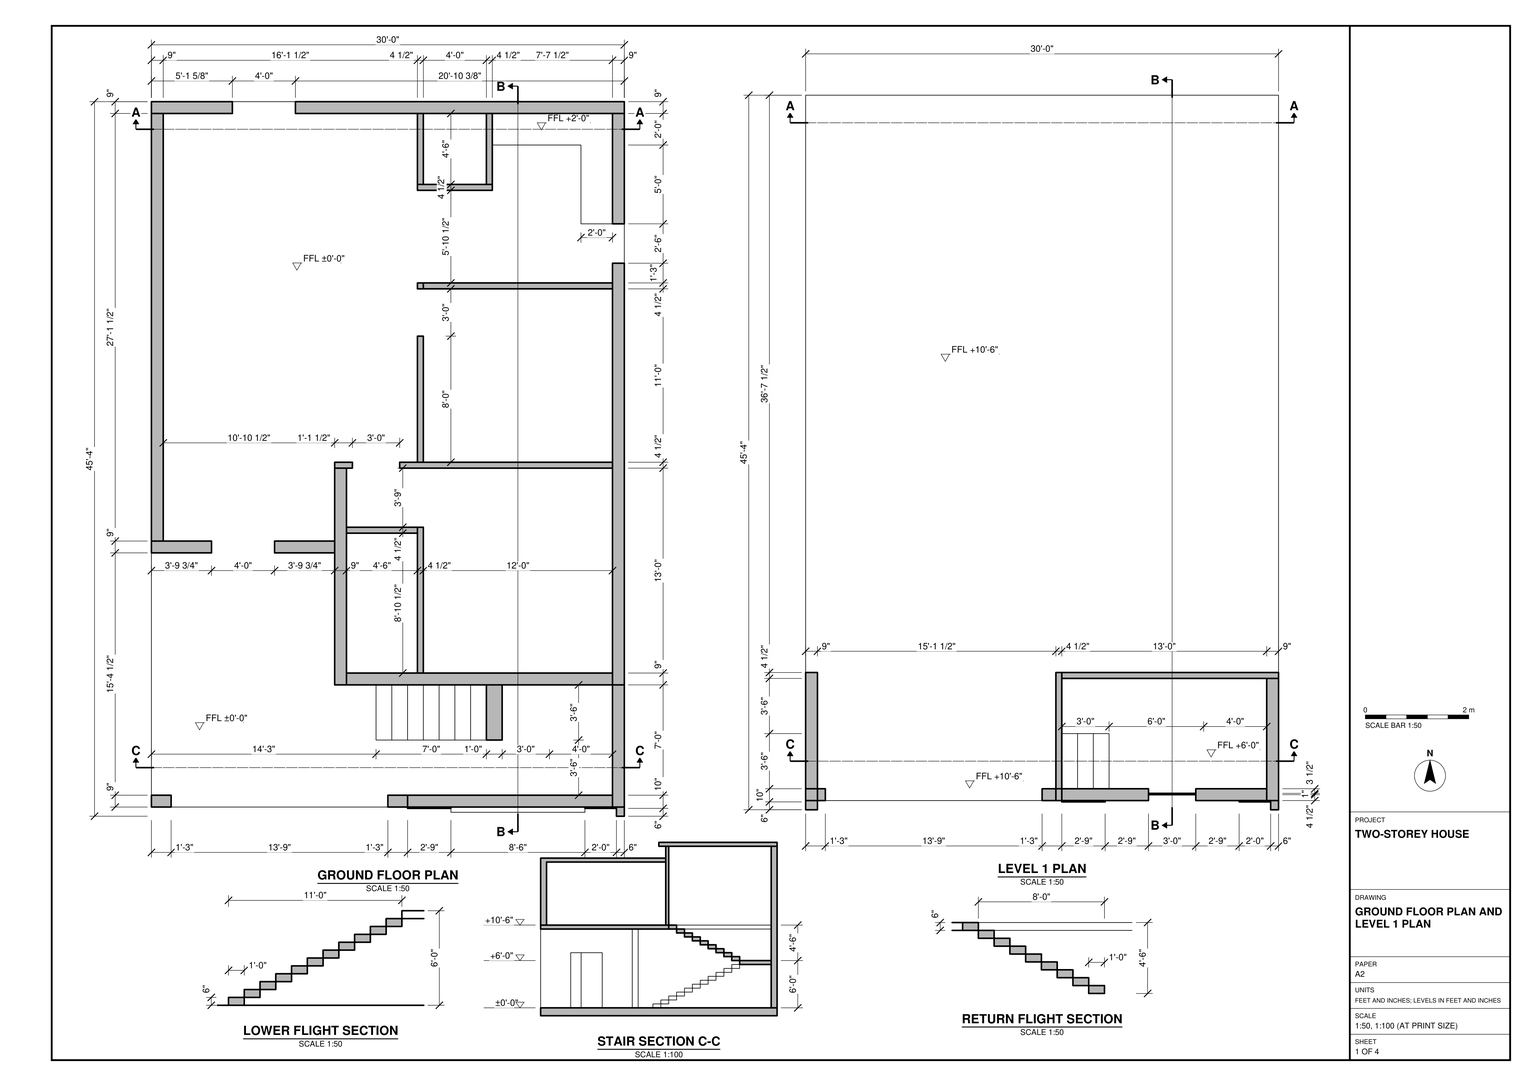
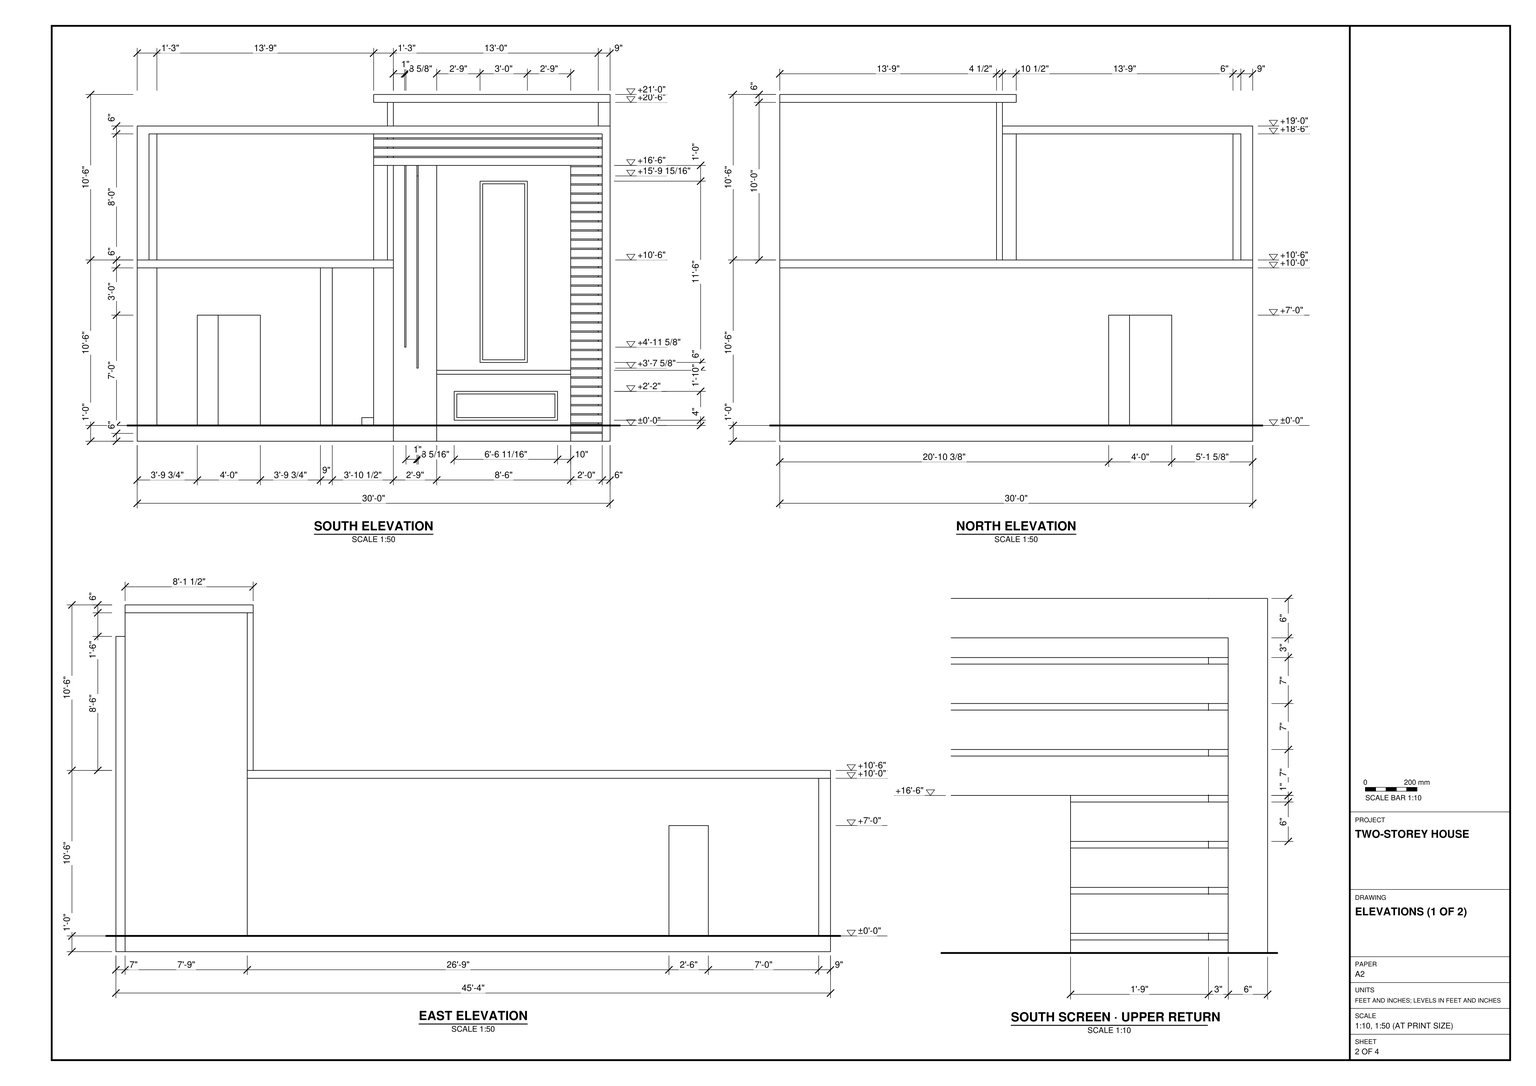
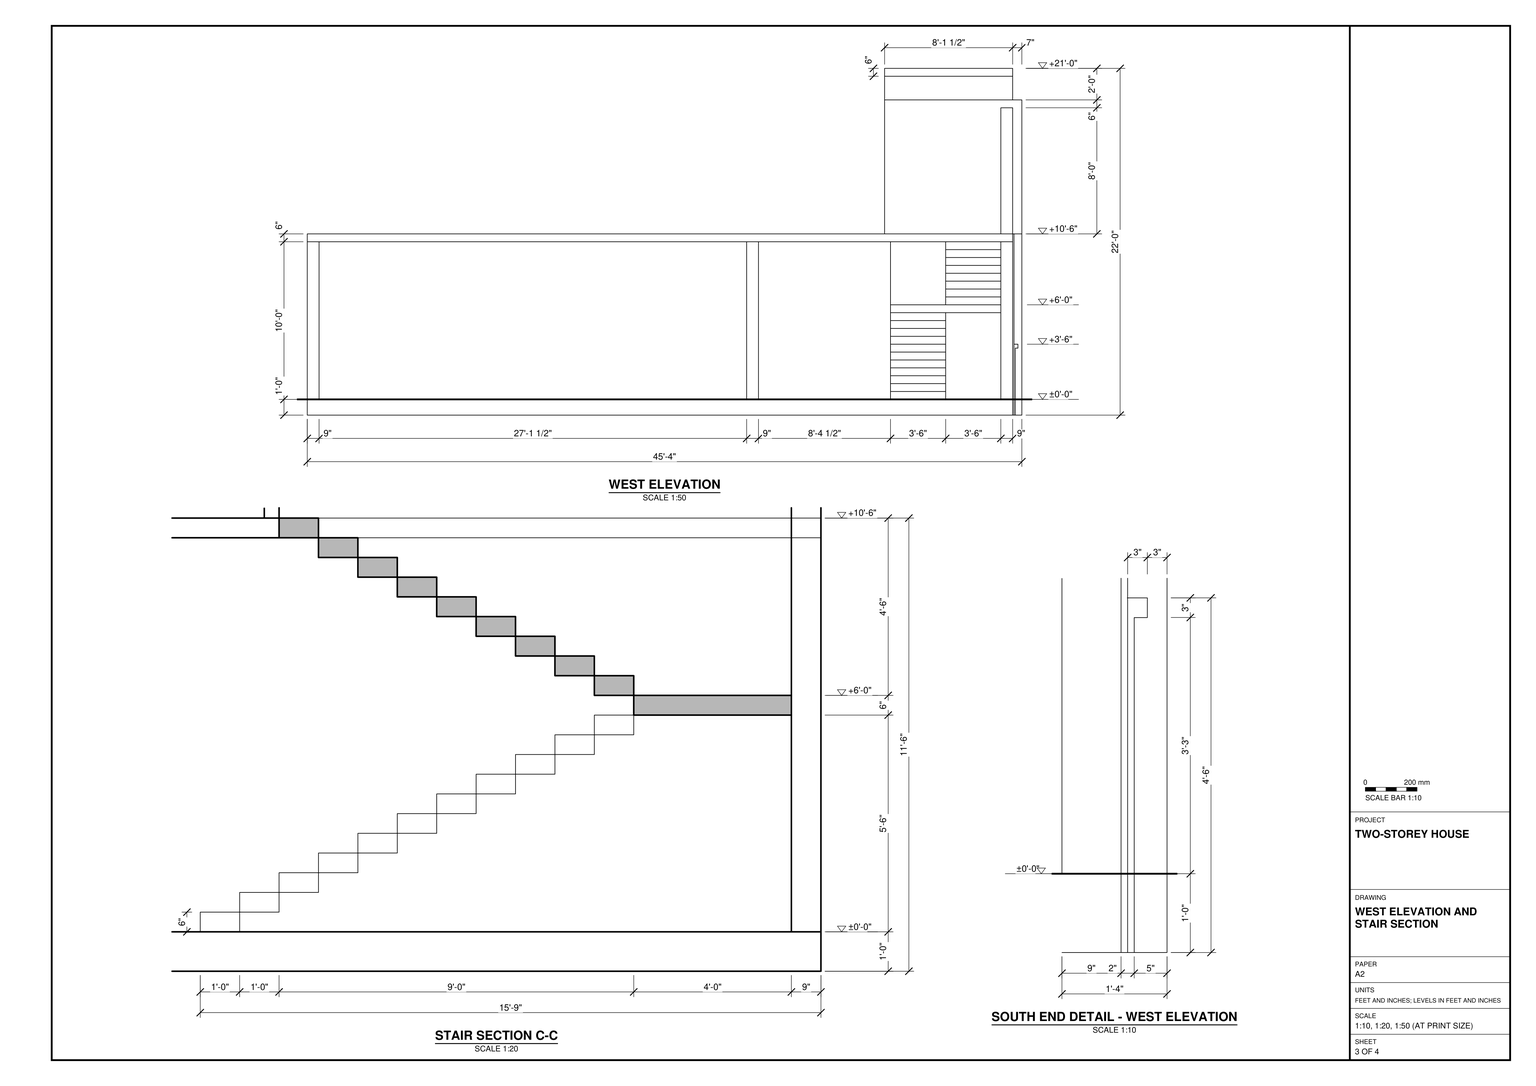
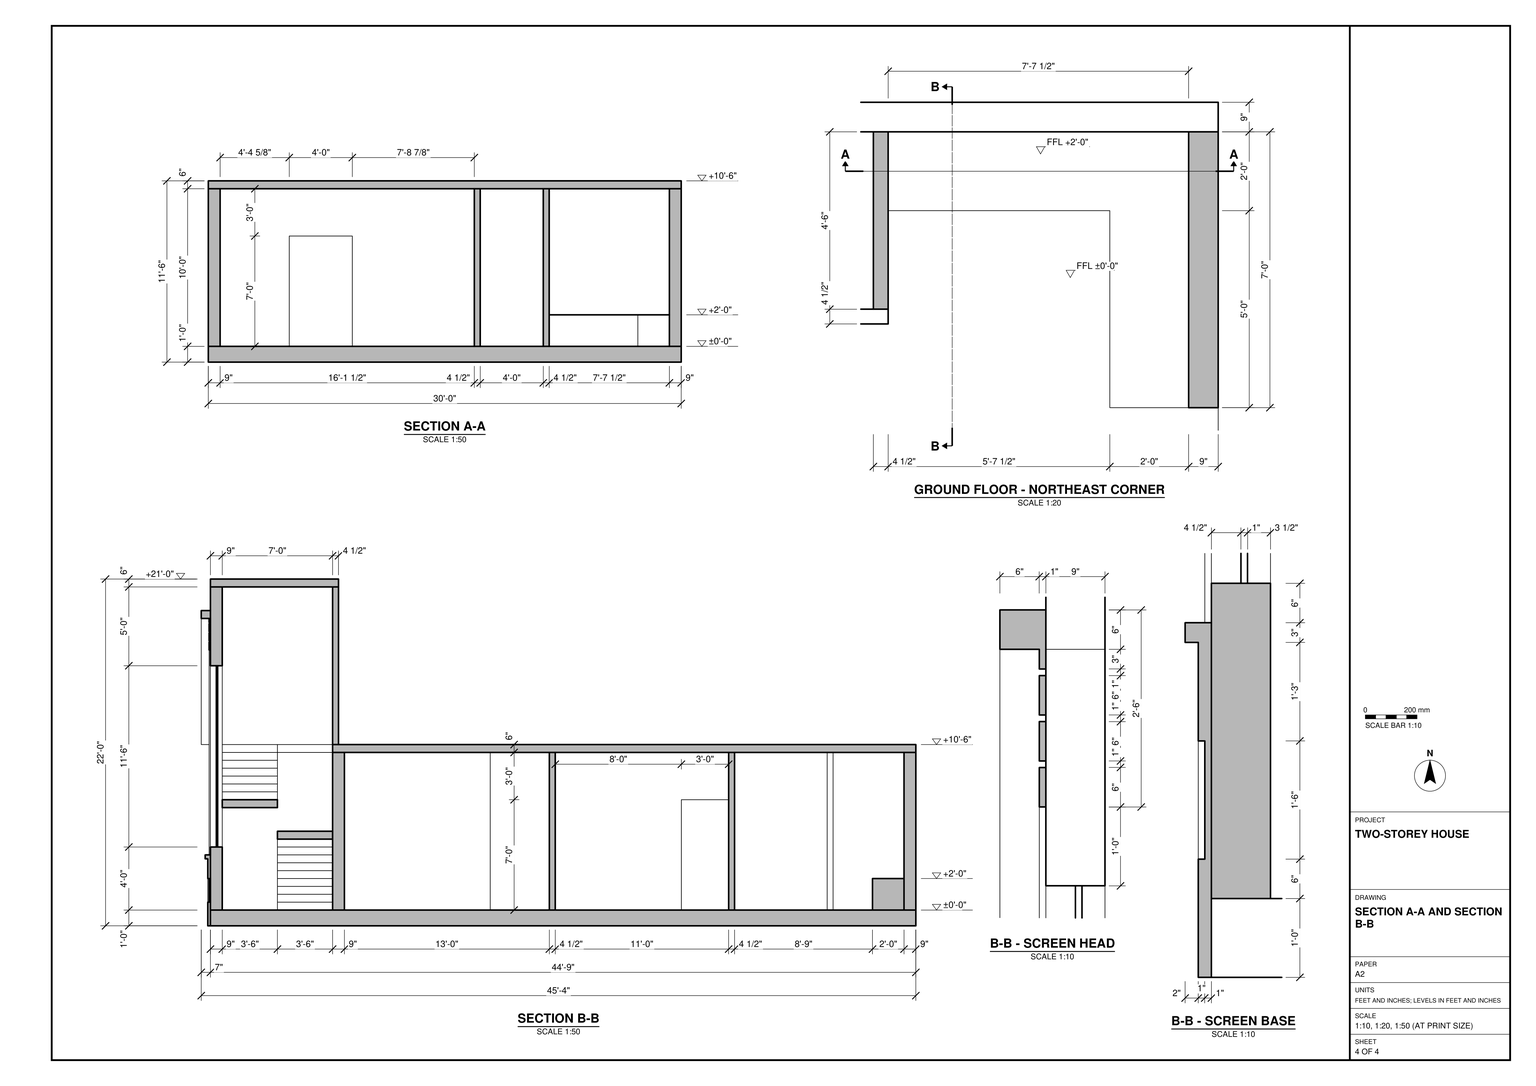
Build the house in SketchUp using task_files/diagram_01.pdf. Work in feet and inches. The house is 30'-0" wide from east to west, 45'-4" deep from north to south and 22'-0" high from the underside of the base slab to the highest roof. Set the ground floor at ±0'-0" and Level 1 at +10'-6".

Follow the ground-floor plan for the recessed south entrance, the large open floor area on the west and the partitions on the east. Use the wall thicknesses shown, distinguishing the 9" walls from the 4 1/2" partitions. Place the door openings at the offsets shown in plan and use the elevations for their heights. Model the base slab and the Level 1 slab, leaving the stair opening at the south end. Build the lower flight up to the +6'-0" landing and reverse direction for the flight to Level 1.

Keep the broad rear portion of Level 1 open and model the stepped flat roofs over the south end. Follow the south elevation for the open bay, the tall narrow frame above the low horizontal panel and the slatted screen that runs up the east edge and across the top. Keep walls, slabs, roofs, and any furniture or joinery pieces in separate groups or components; use components for repeated parts such as screen slats. Any decor or loose items may be suitable library components. Save one SketchUp model as output_files/two_storey_house_with_a_return_stair_and_south_screen.skp.

# SketchUp Ruby script. Lengths in inches.
U = 1.inch
M = Sketchup.active_model
def pt(a) = Geom::Point3d.new(a.map { |v| v * U })
def face(e, loops, mat)
  f = e.add_face(loops[0].map { |a| pt(a) })
  loops[1..].each { |l| e.add_face(l.map { |a| pt(a) }).erase! }
  f.material = f.back_material = mat if mat
  f
end
# faces: each face lists its corners as indices into pts; further lists are holes
def faces(e, pts, list, mat = nil) = list.each { |f| face(e, (f[0].is_a?(Array) ? f : [f]).map { |l| l.map { |i| pts[i] } }, mat) }
# xy, xz, yz: faces in a plane at the given z, y or x. An outline is a flat list of corners, or four numbers for a rectangle; further outlines are holes
def ring(l) = l.size == 4 ? [[l[0], l[1]], [l[2], l[1]], [l[2], l[3]], [l[0], l[3]]] : l.each_slice(2).to_a
def flat(e, list, mat, &to3) = list.each { |f| face(e, (f[0].is_a?(Array) ? f : [f]).map { |l| ring(l).map { |u, v| to3.(u, v) } }, mat) }
def xy(e, z, list, mat = nil) = flat(e, list, mat) { |x, y| [x, y, z] }
def xz(e, y, list, mat = nil) = flat(e, list, mat) { |x, z| [x, y, z] }
def yz(e, x, list, mat = nil) = flat(e, list, mat) { |y, z| [x, y, z] }
def lines(e, pts, list) = list.each { |a, b| e.add_line(pt(pts[a]), pt(pts[b])) }
# prism: a flat outline (further loops are holes) pulled along v
def prism(e, loops, v, mat = nil)
  f = face(e, loops, mat); d = Geom::Vector3d.new(v.map { |x| x * U })
  f.pushpull(f.normal.samedirection?(d) ? d.length : -d.length)
end
def box(e, o, s, mat = nil) = prism(e, [[o, [o[0] + s[0], o[1], o[2]], [o[0] + s[0], o[1] + s[1], o[2]], [o[0], o[1] + s[1], o[2]]]], [0, 0, s[2]], mat)
def at(x, y, z, deg = 0) = Geom::Transformation.translation(pt([x, y, z])) * Geom::Transformation.rotation(ORIGIN, Z_AXIS, deg.degrees)
def axes(o, x, y, z) = Geom::Transformation.new([*x, 0, *y, 0, *z, 0, *pt(o).to_a, 1])
def part(name) = M.definitions.add(name)
# library, detail: a bought-in or finely detailed component or shape, given as its bounding box
def library(name, o, s) = part(name).tap { |d| box(d.entities, o, s) }
def detail(e, o, s) = box(e.add_group.entities, o, s)
def put(e, d, t, mat = nil) = e.add_instance(d, t).tap { |i| i.material = mat if mat }
def group(e, t, mat = nil) = e.add_group.tap { |g| g.transformation = t; g.material = mat if mat }.entities
root = M.entities
M.materials.add("[Color C07]").color = [153, 76, 0]
M.materials.add("[Color E02]").color = [255, 255, 153]
M.materials.add("[Color M00]").color = [255, 255, 255]
M.materials.add("[Color M02]").color = [198, 198, 198]
M.materials.add("[Color M04]").color = [142, 142, 142]
M.materials.add("[Translucent Glass Gray]").color = [128, 128, 128]
M.materials["[Translucent Glass Gray]"].alpha = 0.5
c1 = part("Group\#30")
box(c1.entities,[0,0,0],[15,9,120])
c2 = part("Group\#22")
box(c2.entities,[0,0,0],[12,48,6])
c3 = part("Group\#25")
box(c3.entities,[0,0,0],[12,48,6])
c4 = part("Group\#23")
box(c4.entities,[0,0,0],[12,42,6])
g1 = group(root,at(0,0,-12))
g2 = group(g1,at(0,100,12),"[Color M02]")
box(g2,[0,109.5,0],[9,325.5,120])
g3 = group(g1,at(214.5,401.5,12))
box(g3,[-7.5,0,0],[144,4.5,120])
g4 = group(g1,at(202.5,481,12,-90))
box(g4,[0,0,0],[4.5,57,120])
g5 = group(g1,at(202.5,109,12))
box(g5,[0,0,0],[4.5,111,120])
g6 = group(g1,at(195,6,0),"[Color C07]")
xy(g6,0,[[0,0,33,1]])
xy(g6,210,[[0,0,33,1]])
xz(g6,0,[[0,0,33,0,33,210,18.93,210,18.93,55.65,17.93,55.65,17.93,210,9.62,210,9.62,71.625,8.62,71.625,8.62,210,0,210]])
xz(g6,0,[[17.93,55.65,18.93,201.97],[8.62,71.625,9.62,210],[17.93,201.97,18.93,210]],"[Color M00]")
xz(g6,1,[[0,0,33,210]])
yz(g6,0,[[0,0,1,210]])
yz(g6,33,[[0,0,1,210]])
g7 = group(g1,at(0,100,132),"[Color M02]")
prism(g7,[[[360,444,0],[360,0,0],[195,0,0],[195,-93,0],[0,-93,0],[0,444,0]]],[0,0,6])
g8 = group(g1,at(259.5,451,12))
xy(g8,24,[[67.5,0,91.5,0,91.5,84,0,84,0,60,67.5,60]])
xz(g8,0,[[67.5,0,91.5,24]])
xz(g8,60,[[0,0,67.5,24]])
xz(g8,84,[[0,0,67.5,24],[67.5,0,91.5,24]])
yz(g8,0,[[60,0,84,24]])
yz(g8,67.5,[[0,0,60,24]])
yz(g8,91.5,[[0,0,60,24],[60,0,84,24]])
put(g1,c1,at(0,7,12),"[Color M02]")
g9 = group(g1,at(202.5,269.5,12))
prism(g9,[[[4.5,132,0],[4.5,136.5,0],[4.5,136.5,120],[4.5,0,120],[4.5,0,0],[4.5,96,0],[4.5,96,84],[4.5,132,84]]],[-4.5,0,0])
g10 = group(g1,at(202.5,481,12))
box(g10,[0,0,0],[4.5,54,120])
g11 = group(g1,at(180,7,138),"[Color M02]")
box(g11,[0,0,0],[15,9,96])
g12 = group(g1,at(255,481,12))
box(g12,[0,0,0],[4.5,54,120])
g13 = group(g1,at(139.5,7,12),"[Color M02]")
xy(g13,0,[[55.5,0,211.5,9]])
xy(g13,48,[[121.5,0,157.5,9]])
xy(g13,186,[[121.5,0,157.5,9]])
xy(g13,246,[[55.5,0,211.5,9]])
xz(g13,0,[[[55.5,0,211.5,246],[88.5,42,190.5,198]]])
xz(g13,0,[[[88.5,42,190.5,198],[121.5,48,157.5,186]]],"[Color M04]")
xz(g13,9,[[[55.5,0,211.5,246],[121.5,48,157.5,186]]])
yz(g13,55.5,[[0,0,9,246]])
yz(g13,121.5,[[0,48,9,186]])
yz(g13,157.5,[[0,48,9,186]])
yz(g13,211.5,[[0,0,9,246]])
g14 = group(g13,at(-17.52,4.5,48))
xy(g14,0,[[139.02,0,175.02,1]])
xy(g14,138,[[139.02,0,175.02,1]])
xz(g14,0,[[[139.02,0,175.02,138],[141.02,2,173.02,136]]])
xz(g14,0,[[141.02,2,173.02,136]],"[Translucent Glass Gray]")
xz(g14,1,[[[139.02,0,175.02,138],[141.02,2,173.02,136]]])
xz(g14,1,[[141.02,2,173.02,136]],"[Translucent Glass Gray]")
yz(g14,139.02,[[0,0,1,138]])
yz(g14,175.02,[[0,0,1,138]])
g15 = group(g1,at(228,3,0),"[Color M02]")
g16 = group(g15,at(0,0,0))
xy(g16,0,[[0,2,102,4]])
xy(g16,18,[[15.31,2,90,3]])
xy(g16,36,[[15.31,2,90,3]])
xy(g16,51,[[0,0,102,2]])
xy(g16,54,[[0,0,102,4]],"[Color M00]")
xz(g16,0,[[0,51,102,54]],"[Color M00]")
xz(g16,2,[[[13.31,16,92,38],[15.31,18,90,36]]],"[Color M00]")
xz(g16,2,[[[0,0,102,51],[13.31,16,92,38]]],"[Color M04]")
xz(g16,3,[[15.31,18,90,36]],"[Color C07]")
xz(g16,4,[[0,0,102,54]])
yz(g16,0,[[2,0,2,51,0,51,0,54,4,54,4,0]])
yz(g16,15.31,[[2,18,3,36]])
yz(g16,90,[[2,18,3,36]])
yz(g16,102,[[2,0,4,0,4,54,0,54,0,51,2,51]])
g17 = group(g1,at(330,6,0),"[Color M02]")
xy(g17,0,[[24,-6,24,0,0,0,0,1,30,1,30,-6]])
xy(g17,6,[[0,0,24,1]])
xy(g17,7,[[0,0,24,1]])
xy(g17,13,[[0,0,24,1]])
xy(g17,14,[[0,0,24,1]])
xy(g17,20,[[0,0,24,1]])
xy(g17,21,[[0,0,24,1]])
xy(g17,27,[[0,0,24,1]])
xy(g17,28,[[0,0,24,1]])
xy(g17,34,[[0,0,24,1]])
xy(g17,35,[[0,0,24,1]])
xy(g17,41,[[0,0,24,1]])
xy(g17,42,[[0,0,24,1]])
xy(g17,48,[[0,0,24,1]])
xy(g17,49,[[0,0,24,1]])
xy(g17,55,[[0,0,24,1]])
xy(g17,56,[[0,0,24,1]])
xy(g17,62,[[0,0,24,1]])
xy(g17,63,[[0,0,24,1]])
xy(g17,69,[[0,0,24,1]])
xy(g17,70,[[0,0,24,1]])
xy(g17,76,[[0,0,24,1]])
xy(g17,77,[[0,0,24,1]])
xy(g17,83,[[0,0,24,1]])
xy(g17,84,[[0,0,24,1]])
xy(g17,90,[[0,0,24,1]])
xy(g17,91,[[0,0,24,1]])
xy(g17,97,[[0,0,24,1]])
xy(g17,98,[[0,0,24,1]])
xy(g17,104,[[0,0,24,1]])
xy(g17,105,[[0,0,24,1]])
xy(g17,111,[[0,0,24,1]])
xy(g17,112,[[0,0,24,1]])
xy(g17,118,[[0,0,24,1]])
xy(g17,119,[[0,0,24,1]])
xy(g17,125,[[0,0,24,1]])
xy(g17,126,[[0,0,24,1]])
xy(g17,132,[[0,0,24,1]])
xy(g17,133,[[0,0,24,1]])
xy(g17,138,[[-330,-6,-321,98.5]])
xy(g17,139,[[0,0,24,1]])
xy(g17,140,[[0,0,24,1]])
xy(g17,146,[[0,0,24,1]])
xy(g17,147,[[0,0,24,1]])
xy(g17,153,[[0,0,24,1]])
xy(g17,154,[[0,0,24,1]])
xy(g17,160,[[0,0,24,1]])
xy(g17,161,[[0,0,24,1]])
xy(g17,167,[[0,0,24,1]])
xy(g17,168,[[0,0,24,1]])
xy(g17,174,[[0,0,24,1]])
xy(g17,175,[[0,0,24,1]])
xy(g17,181,[[0,0,24,1]])
xy(g17,182,[[0,0,24,1]])
xy(g17,188,[[0,0,24,1]])
xy(g17,189,[[0,0,24,1]])
xy(g17,195,[[0,0,24,1]])
xy(g17,196,[[0,0,24,1]])
xy(g17,202,[[0,0,24,1]])
xy(g17,203,[[0,0,24,1]],"[Color E02]")
xy(g17,209,[[0,0,24,1]])
xy(g17,210,[[-150,0,0,1],[0,0,24,1]])
xy(g17,216,[[-150,0,24,1]])
xy(g17,217,[[-150,0,24,1]])
xy(g17,223,[[-150,0,24,1]])
xy(g17,224,[[-150,0,24,1]])
xy(g17,230,[[-150,0,24,1]])
xy(g17,231,[[-150,0,24,1]])
xy(g17,234,[[-321,-6,-321,98.5,-150,98.5,-150,0,24,0,24,-6],[-150,1,-139.5,98.5]])
xy(g17,240,[[-330,-6,30,-6,30,1,-139.5,1,-139.5,98.5,-330,98.5]])
xz(g17,-6,[[24,0,30,0,30,240,-330,240,-330,138,-321,138,-321,234,24,234]])
xz(g17,0,[[0,0,24,6],[0,7,24,13],[0,14,24,20],[0,21,24,27],[0,28,24,34],
  [0,35,24,41],[0,42,24,48],[0,49,24,55],[0,56,24,62],[0,63,24,69],
  [0,70,24,76],[0,77,24,83],[0,84,24,90],[0,91,24,97],[0,98,24,104],
  [0,105,24,111],[0,112,24,118],[0,119,24,125],[0,126,24,132],[0,133,24,139],
  [0,140,24,146],[0,147,24,153],[0,154,24,160],[0,161,24,167],[0,168,24,174],
  [0,175,24,181],[0,182,24,188],[0,189,24,195],[0,196,24,202],[0,203,24,209],
  [-150,210,24,216],[-150,217,24,223],[-150,224,24,230],[-150,231,24,234]],"[Color E02]")
xz(g17,1,[[0,0,0,6,24,6,24,7,0,7,0,13,24,13,24,14,0,14,0,20,24,20,24,21,0,21,0,27,24,27,24,28,0,28,0,34,24,34,24,35,0,35,0,41,24,41,24,42,0,42,0,48,24,48,24,49,0,49,0,55,24,55,24,56,0,56,0,62,24,62,24,63,0,63,0,69,24,69,24,70,0,70,0,76,24,76,24,77,0,77,0,83,24,83,24,84,0,84,0,90,24,90,24,91,0,91,0,97,24,97,24,98,0,98,0,104,24,104,24,105,0,105,0,111,24,111,24,112,0,112,0,118,24,118,24,119,0,119,0,125,24,125,24,126,0,126,0,132,24,132,24,133,0,133,0,139,24,139,24,140,0,140,0,146,24,146,24,147,0,147,0,153,24,153,24,154,0,154,0,160,24,160,24,161,0,161,0,167,24,167,24,168,0,168,0,174,24,174,24,175,0,175,0,181,24,181,24,182,0,182,0,188,24,188,24,189,0,189,0,195,24,195,24,196,0,196,0,202,24,202,24,203,0,203,0,209,24,209,24,210,-150,210,-150,216,24,216,24,217,-150,217,-150,223,24,223,24,224,-150,224,-150,230,24,230,24,231,-150,231,-150,234,0,234,0,240,30,240,30,0],[-139.5,234,0,240]])
xz(g17,98.5,[[-330,138,-330,240,-139.5,240,-139.5,234,-321,234,-321,138]])
yz(g17,-330,[[-6,138,98.5,240]])
yz(g17,-321,[[-6,138,98.5,234]])
yz(g17,-150,[[0,210,1,216],[0,217,1,223],[0,224,1,230],[0,231,1,234]])
yz(g17,-139.5,[[1,234,98.5,240]])
yz(g17,0,[[0,0,1,6],[0,7,1,13],[0,14,1,20],[0,21,1,27],[0,28,1,34],
  [0,35,1,41],[0,42,1,48],[0,49,1,55],[0,56,1,62],[0,63,1,69],
  [0,70,1,76],[0,77,1,83],[0,84,1,90],[0,91,1,97],[0,98,1,104],
  [0,105,1,111],[0,112,1,118],[0,119,1,125],[0,126,1,132],[0,133,1,139],
  [0,140,1,146],[0,147,1,153],[0,154,1,160],[0,161,1,167],[0,168,1,174],
  [0,175,1,181],[0,182,1,188],[0,189,1,195],[0,196,1,202],[0,203,1,209]])
yz(g17,24,[[-6,0,-6,234,0,234,0,231,1,231,1,230,0,230,0,224,1,224,1,223,0,223,0,217,1,217,1,216,0,216,0,210,1,210,1,209,0,209,0,203,1,203,1,202,0,202,0,196,1,196,1,195,0,195,0,189,1,189,1,188,0,188,0,182,1,182,1,181,0,181,0,175,1,175,1,174,0,174,0,168,1,168,1,167,0,167,0,161,1,161,1,160,0,160,0,154,1,154,1,153,0,153,0,147,1,147,1,146,0,146,0,140,1,140,1,139,0,139,0,133,1,133,1,132,0,132,0,126,1,126,1,125,0,125,0,119,1,119,1,118,0,118,0,112,1,112,1,111,0,111,0,105,1,105,1,104,0,104,0,98,1,98,1,97,0,97,0,91,1,91,1,90,0,90,0,84,1,84,1,83,0,83,0,77,1,77,1,76,0,76,0,70,1,70,1,69,0,69,0,63,1,63,1,62,0,62,0,56,1,56,1,55,0,55,0,49,1,49,1,48,0,48,0,42,1,42,1,41,0,41,0,35,1,35,1,34,0,34,0,28,1,28,1,27,0,27,0,21,1,21,1,20,0,20,0,14,1,14,1,13,0,13,0,7,1,7,1,6,0,6,0,0]])
yz(g17,30,[[-6,0,1,240]])
p = [[-139.5,1,240],[-139.5,1,240.125]]
lines(g17,p,[[0,1]])
g18 = group(g1,at(0,535,12),"[Color M02]")
prism(g18,[[[0,0,0],[61.625,0,0],[61.625,0,84],[109.625,0,84],[109.625,0,0],[360,0,0],[360,0,120],[0,0,120]]],[0,9,0])
g19 = group(g1,at(148.5,215.5,12))
box(g19,[0,0,0],[54,4.5,120])
g20 = group(g1,at(0,7,138),"[Color M02]")
box(g20,[0,0,0],[15,9,96])
put(g1,c1,at(180,7,12),"[Color M02]")
g21 = group(g1,at(351,109,12),"[Color M02]")
prism(g21,[[[9,342,0],[9,426,0],[9,426,120],[9,-9,120],[9,-9,0],[9,312,0],[9,312,84],[9,342,84]]],[-9,0,0])
g22 = group(g1,at(190.5,7,258),"[Color M02]")
box(g22,[-10.5,0,0],[180,97.5,6])
g23 = group(g1,at(190.5,7,138))
xy(g23,0,[[0,0,4.5,93],[0,93,4.5,97.5],[4.5,93,169.5,97.5]])
xy(g23,120,[[0,0,4.5,97.5],[4.5,93,169.5,97.5]])
xz(g23,0,[[0,0,4.5,120]])
xz(g23,93,[[4.5,0,169.5,120]])
xz(g23,97.5,[[0,0,4.5,120],[4.5,0,169.5,120]])
yz(g23,0,[[0,0,97.5,120]])
yz(g23,4.5,[[0,0,93,120],[93,0,97.5,120]])
yz(g23,169.5,[[93,0,97.5,120]])
g24 = group(g1,at(148.5,265,12))
prism(g24,[[[-9,0,0],[4.5,0,0],[4.5,0,84],[40.5,0,84],[40.5,0,0],[202.5,0,0],[202.5,0,120],[-9,0,120]]],[0,4.5,0])
g25 = group(g1,at(351,16,12),"[Color M02]")
box(g25,[0,-9,0],[9,93,246])
g26 = group(g1,at(9,200.5,12),"[Color M02]")
prism(g26,[[[36.75,9,0],[-9,9,0],[-9,9,120],[130.5,9,120],[130.5,9,0],[84.75,9,0],[84.75,9,84],[36.75,9,84]]],[0,-9,0])
g27 = group(g1,at(0,100,-12),"[Color M02]")
prism(g27,[[[360,444,12],[360,-93,12],[195,-93,12],[0,-93,12],[0,444,12]]],[0,0,12])
g28 = group(g1,at(171,52,12))
put(g28,c2,axes([36,6,18],[1,0,0],[0,0.875,0],[0,0,1]))
put(g28,c2,axes([48,6,24],[1,0,0],[0,0.875,0],[0,0,1]))
put(g28,c2,axes([24,6,12],[1,0,0],[0,0.875,0],[0,0,1]))
put(g28,c2,axes([84,6,42],[1,0,0],[0,0.875,0],[0,0,1]))
put(g28,c3,axes([108,6,54],[1,0,0],[0,0.875,0],[0,0,1]))
put(g28,c2,axes([60,6,30],[1,0,0],[0,0.875,0],[0,0,1]))
put(g28,c2,axes([72,6,36],[1,0,0],[0,0.875,0],[0,0,1]))
put(g28,c2,axes([0,6,0],[1,0,0],[0,0.875,0],[0,0,1]))
put(g28,c2,axes([12,6,6],[1,0,0],[0,0.875,0],[0,0,1]))
put(g28,c2,axes([96,6,48],[1,0,0],[0,0.875,0],[0,0,1]))
put(g28,c3,axes([120,6,60],[1,0,0],[0,0.875,0],[0,0,1]))
g29 = group(g28,at(132,0,66))
box(g29,[0,-36,0],[48,84,6])
put(g28,c4,at(120,-36,72))
put(g28,c4,at(108,-36,78))
put(g28,c4,at(96,-36,84))
put(g28,c4,at(84,-36,90))
put(g28,c4,at(72,-36,96))
put(g28,c4,at(60,-36,102))
put(g28,c4,at(48,-36,108))
put(g28,c4,at(36,-36,114))
put(g28,c4,at(24,-36,120))
g30 = group(g1,at(139.5,100,12),"[Color M02]")
box(g30,[0,0,0],[9,165,120])
g31 = group(g1,at(144,100,12),"[Color M02]")
box(g31,[4.5,0,0],[202.5,9,120])
